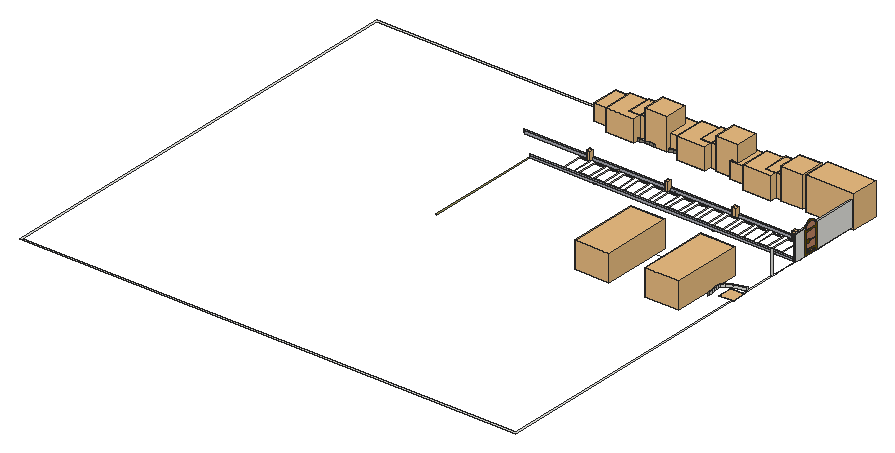
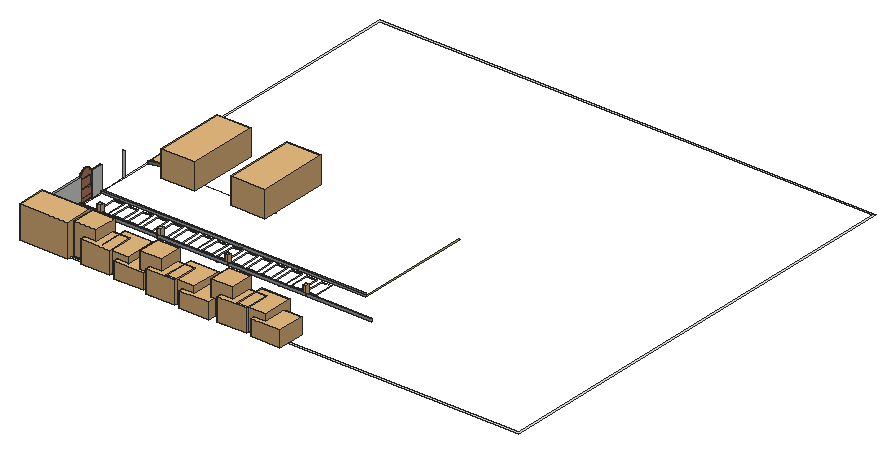
# SketchUp Ruby script. Lengths in inches.
U = 1.inch
M = Sketchup.active_model
def pt(a) = Geom::Point3d.new(a.map { |v| v * U })
def face(e, loops, mat)
  f = e.add_face(loops[0].map { |a| pt(a) })
  loops[1..].each { |l| e.add_face(l.map { |a| pt(a) }).erase! }
  f.material = f.back_material = mat if mat
  f
end
# faces: each face lists its corners as indices into pts; further lists are holes
def faces(e, pts, list, mat = nil) = list.each { |f| face(e, (f[0].is_a?(Array) ? f : [f]).map { |l| l.map { |i| pts[i] } }, mat) }
# xy, xz, yz: faces in a plane at the given z, y or x. An outline is a flat list of corners, or four numbers for a rectangle; further outlines are holes
def ring(l) = l.size == 4 ? [[l[0], l[1]], [l[2], l[1]], [l[2], l[3]], [l[0], l[3]]] : l.each_slice(2).to_a
def flat(e, list, mat, &to3) = list.each { |f| face(e, (f[0].is_a?(Array) ? f : [f]).map { |l| ring(l).map { |u, v| to3.(u, v) } }, mat) }
def xy(e, z, list, mat = nil) = flat(e, list, mat) { |x, y| [x, y, z] }
def xz(e, y, list, mat = nil) = flat(e, list, mat) { |x, z| [x, y, z] }
def yz(e, x, list, mat = nil) = flat(e, list, mat) { |y, z| [x, y, z] }
def lines(e, pts, list) = list.each { |a, b| e.add_line(pt(pts[a]), pt(pts[b])) }
# prism: a flat outline (further loops are holes) pulled along v
def prism(e, loops, v, mat = nil)
  f = face(e, loops, mat); d = Geom::Vector3d.new(v.map { |x| x * U })
  f.pushpull(f.normal.samedirection?(d) ? d.length : -d.length)
end
def box(e, o, s, mat = nil) = prism(e, [[o, [o[0] + s[0], o[1], o[2]], [o[0] + s[0], o[1] + s[1], o[2]], [o[0], o[1] + s[1], o[2]]]], [0, 0, s[2]], mat)
def at(x, y, z, deg = 0) = Geom::Transformation.translation(pt([x, y, z])) * Geom::Transformation.rotation(ORIGIN, Z_AXIS, deg.degrees)
def axes(o, x, y, z) = Geom::Transformation.new([*x, 0, *y, 0, *z, 0, *pt(o).to_a, 1])
def part(name) = M.definitions.add(name)
# library, detail: a bought-in or finely detailed component or shape, given as its bounding box
def library(name, o, s) = part(name).tap { |d| box(d.entities, o, s) }
def detail(e, o, s) = box(e.add_group.entities, o, s)
def put(e, d, t, mat = nil) = e.add_instance(d, t).tap { |i| i.material = mat if mat }
def group(e, t, mat = nil) = e.add_group.tap { |g| g.transformation = t; g.material = mat if mat }.entities
root = M.entities
M.materials.add("Marble_01_1K").color = [230, 221, 211]
M.materials.add("Marble_20_1K").color = [172, 173, 182]
M.materials.add("Material__4").color = [36, 36, 36]
M.materials.add("Material__6").color = [79, 108, 5]
M.materials.add("Plaster_06_1K").color = [141, 135, 122]
M.materials.add("Soil_04_1K").color = [152, 146, 88]
M.materials.add("[Color D08]").color = [102, 76, 0]
M.materials.add("[Modern Siding]").color = [191, 132, 100]
M.materials.add("calathea lutea").color = [121, 145, 80]
c1 = library("Group\#54",[0,0,0],[2062.46,2062.46,4833.66])
c2 = part("Landscape+Light")
put(c2.entities,c1,at(-2096.57,-1031.23,-3775.98))
c3 = library("ew",[-14.92,-16.84,0],[29.84,33.68,0.01])
c4 = part("Group\#156")
g1 = group(c4.entities,at(8.61,38.85,0))
xy(g1,0,[[0,0,2.82,19.1,22.58,0],[22.58,0,2.82,19.1,22.58,19.1]],"calathea lutea")
p = [[2.82,19.1,0],[7.19,48.22,5.13],[10.77,48.22,5.13],[12.74,48.22,5.13],[22.58,48.22,5.13],[22.58,19.1,0]]
faces(g1,p,[[0,1,2,3,4,5]],"calathea lutea")
g2 = group(c4.entities,at(-0.77,-7.77,0))
p = [[14.8125,23.31,1.46],[21.35,23.31,0],[14.8125,0,1.46],[21.35,0,0],[27.89,0,1.46],[27.89,23.31,1.46],
  [8.27,46.62,2.92],[21.35,46.62,0],[34.4375,46.62,2.92],[4.47,23.31,6.43],[0,0,8.59],[33.76,0,4.28],
  [33.76,23.31,4.28]]
faces(g2,p,[[0,1,2],[3,2,1],[4,3,5],[1,5,3],[6,7,0],[1,0,7],[5,1,8],[7,8,1],
  [9,0,2,10],[11,4,5,12],[9,6,0],[12,5,8]],"calathea lutea")
c5 = part("Group\#150")
xy(c5.entities,0,[[0,0,0,33.87,27.21,33.87,19.71,0]],"calathea lutea")
c6 = part("Group\#157")
xy(c6.entities,1.04,[[21.13,33.87,21.13,57.59,32.375,57.59,27.12,33.87]],"calathea lutea")
xy(c6.entities,1.32,[[0.12,33.87,7.74,57.59]],"calathea lutea")
p = [[7.74,33.87,1.32],[11.8,57.59,0.61],[15.24,57.59,0],[15.24,33.87,0],[18.43,57.59,0.5625],[21.13,57.59,1.04],
  [21.13,33.87,1.04],[15.24,77.7,2.36],[21.13,77.7,3.4],[7.74,57.59,1.32],[7.74,77.7,3.69],[36.83,77.7,3.4],
  [32.375,57.59,1.04],[0.12,57.59,1.32],[0.12,77.7,3.69]]
faces(c6.entities,p,[[0,1,2,3],[3,2,4],[3,4,5,6],[7,2,1],[8,4,2,7],[0,9,1],[7,1,9,10],[8,5,4],
  [11,12,5,8],[10,9,13,14]],"calathea lutea")
put(c6.entities,c5,axes([0,-16.9375,0],[1,0,0],[0,1.5,0],[0,0,1]))
c7 = part("Group\#155")
g3 = group(c7.entities,at(0,-17.3,0))
xy(g3,0,[[0,0,28.07,51.9]],"calathea lutea")
g4 = group(c7.entities,at(0.9,34.6,0))
xy(g4,0,[[13.14,0,13.14,26.22,16.85,26.22],[13.14,0,16.85,26.22,20.16,26.22,20.16,0]],"calathea lutea")
p = [[6.36,0,1.82],[9.95,26.22,0.86],[13.14,26.22,0],[13.14,0,0],[20.16,0,0],[20.16,26.22,0],
  [27.07,26.22,1.22],[27.07,0,1.22],[13.14,49.5625,5.91],[20.16,49.5625,5.91],[16.85,26.22,0],[27.07,49.5625,7.125],
  [6.36,26.22,1.82],[6.36,49.5625,7.72],[0,0,4.78],[0,26.22,4.78],[0,49.5625,10.6875]]
faces(g4,p,[[0,1,2,3],[4,5,6,7],[8,2,1],[9,10,2,8],[9,5,10],[11,6,5,9],[0,12,1],[8,1,12,13],
  [14,15,12,0],[13,12,15,16]],"calathea lutea")
c8 = part("Group\#154")
put(c8.entities,c5,axes([0,-16.9375,0],[1,0,0],[0,1.5,0],[0,0,1]))
g5 = group(c8.entities,at(-0.23,33.4,-0.35))
p = [[15.12,39.14,-19.87],[15.12,20.54,-11.86],[11.68,20.84,-11.33],[21.02,39.66,-18.97],[18.3125,20.82,-11.37],[7.62,21.2,-10.71],
  [7.62,39.8,-18.72],[21.02,21.06,-10.96],[36.72,39.66,-18.97],[32.26,21.06,-10.96],[0,21.2,-10.71],[0,39.8,-18.72],
  [7.62,0.66,1.15],[15.12,0,0],[21.02,0.52,0.9],[27.01,0.52,0.9],[0,0.66,1.15]]
faces(g5,p,[[0,1,2],[3,4,1,0],[0,2,5,6],[3,7,4],[8,9,7,3],[6,5,10,11],[12,2,1,13],[13,1,4],
  [13,4,7,14],[12,5,2],[14,7,9,15],[16,10,5,12]],"calathea lutea")
c9 = part("Foliage cluster")
put(c9.entities,c4,axes([37.24,8.07,75.17],[1,0,0],[0,0.45554,-0.89021],[0,0.89021,0.45554]))
put(c9.entities,c6,axes([69.44,65.48,16.68],[-0.53288,-0.84619,0],[0.14694,-0.09253,0.98481],[-0.83334,0.52478,0.17365]))
put(c9.entities,c7,axes([47.9375,70.43,17.04],[0.74664,-0.66523,0],[0.11552,0.12965,0.98481],[-0.65512,-0.7353,0.17365]))
put(c9.entities,c4,axes([76.19,10.66,75.17],[0.70711,0.70711,0],[-0.32212,0.32212,-0.89021],[-0.62948,0.62948,0.45554]))
put(c9.entities,c4,axes([101.91,40.03,75.17],[0,1,0],[-0.45554,0,-0.89021],[-0.89021,0,0.45554]))
put(c9.entities,c4,axes([99.32,78.99,75.17],[-0.70711,0.70711,0],[-0.32212,-0.32212,-0.89021],[-0.62948,-0.62948,0.45554]))
put(c9.entities,c7,axes([34.81,63.36,17.04],[0.99956,-0.02967,0],[0.00515,0.17357,0.98481],[-0.02922,-0.98437,0.17365]))
put(c9.entities,c7,axes([48,37.4,15.8],[-0.14436,0.98953,0],[-0.40248,-0.05871,0.91355],[0.90398,0.13188,0.40674]))
put(c9.entities,c6,axes([56.87,39.77,12.28],[-0.67695,0.4263,0],[-0.18016,-0.28609,0.72505],[0.38636,0.61353,0.33809]))
put(c9.entities,c6,axes([36.12,43.25,12.28],[0.18947,0.77724,0],[-0.32848,0.08007,0.72505],[0.70442,-0.17172,0.33809]))
put(c9.entities,c8,axes([35.1,54.93,11.375],[0.79719,0.06694,0],[-0.03636,0.43302,0.6717],[0.05621,-0.66934,0.43454]))
put(c9.entities,c6,axes([41.66,47.32,12.28],[0.45082,0.66088,0],[-0.2793,0.19053,0.72505],[0.59896,-0.40858,0.33809]))
put(c9.entities,c6,axes([47.89,59.4,12.28],[0.79719,0.06694,0],[-0.02829,0.33691,0.72505],[0.06067,-0.7225,0.33809]))
put(c9.entities,c8,axes([29.53,49.96,11.375],[0.65692,0.45657,0],[-0.248,0.35682,0.6717],[0.38335,-0.55156,0.43454]))
put(c9.entities,c8,axes([29.9,49.27,12.86],[0.34062,0.72386,0],[-0.22849,0.10752,0.7591],[0.68685,-0.32321,0.25252]))
put(c9.entities,c8,axes([36.33,48.82,8.99],[0.09232,0.62522,0],[-0.3396,0.05015,0.53064],[0.52495,-0.07752,0.34329]))
put(c9.entities,c8,axes([49.82,38.52,8.99],[-0.54622,0.31791,0],[-0.17268,-0.29669,0.53064],[0.26692,0.45862,0.34329]))
put(c9.entities,c8,axes([55.68,39.21,8.99],[-0.632,0.00221,0],[-0.0012,-0.34328,0.53064],[0.00185,0.53064,0.34329]))
c10 = library("Group\#28",[0,0,0],[86.94,78.77,46.4375])
c11 = library("Group\#14",[-978.71,-103.24,719.12],[90.2,76.4,68.29])
c12 = library("Group\#13",[-906.16,-138.28,686.8],[98.25,106.18,75.79])
c13 = library("Group\#202",[-3.47,-2.45,12.47],[53.14,54.93,75.51])
c14 = part("Group\#35")
put(c14.entities,c9,axes([161.54,39.59,6.01],[0.19523,-0.19694,0],[0.19694,0.19523,0],[0,0,0.24957]))
put(c14.entities,c10,axes([0,18.48,0.92],[0.83,0,0],[0,0.83,0],[0,0,0.83]))
put(c14.entities,c11,axes([859.63,98.87,-568.1],[0.79,0,0],[0,0.79,0],[0,0,0.79]),"Material__4")
put(c14.entities,c12,axes([669.69,95.42,-472.48],[0.69,0,0],[0,0.69,0],[0,0,0.69]),"Material__6")
put(c14.entities,c13,at(133.52,12.51,-9.6))
c15 = library("t1",[-17.79,-17.21,0],[35.58,34.42,0.01])
c16 = library("light",[-4,-4,0],[8,8,0.01])
c17 = library("tt",[-12.4,-12.1,0],[24.8,24.2,0.01])
c18 = library("Evoque+Azul+Marinho+As+Novinha+Fica+Loca+2017",[-10.19,-69.08,0],[168.96,82.02,63.04])
c19 = library("Group\#32",[86.45,10.0625,0],[116.41,67.6,78.39])
box(root,[1204.46,846.16,0],[4,28.07,60])
xy(root,0,[[8.46,0.95,8.46,1080.74,1208.46,1080.74,1208.46,918.16,1207.93,910.21,1204.99,910.21,1204.46,918.16,1204.46,1076.74,12.46,1076.74,12.46,4.95,1204.46,4.95,1204.46,703.68,1204.54,706.84,1204.46,706.82,1204.46,777.17,1208.46,777.17,1208.46,0.95],[1204.46,703.68,1204.46,706.82,1204.54,706.84],[1202.44,846.16,1202.44,918.16,1204.46,918.16,1204.46,910.21,1204.99,910.21,1206.46,888.16,1207.93,910.21,1206.46,888.16,1204.46,858.17,1205.06,846.16],[1202.44,846.16,1202.44,918.16,1204.46,918.16,1204.46,910.21,1204.99,910.21,1206.46,888.16,1208.46,858.17,1208.46,918.16,1206.46,888.16,1204.46,858.17,1205.06,846.16],[1205.06,846.16,1207.87,846.16,1208.46,858.17,1204.46,858.17],
  [1207.87,846.16,1208.46,846.16,1208.46,858.17],[1204.46,858.17,1206.46,888.16,1208.46,858.17],[1208.46,858.17,1206.46,888.16,1207.93,910.21,1208.46,910.21],[1206.46,888.16,1204.99,910.21,1207.93,910.21],[1204.46,910.21,1204.46,918.16,1204.99,910.21],
  [1207.93,910.21,1208.46,918.16,1208.46,910.21]])
xy(root,0,[[561.69,565.82,561.69,850.66,1202.44,850.66,1202.44,846.16,566.19,846.16,566.19,565.82]],"Soil_04_1K")
xz(root,777.17,[[1204.46,0,1208.46,60]])
xz(root,846.16,[[566.19,0,870.83,6],[870.83,0,1202.44,6]],"Marble_20_1K")
xz(root,850.66,[[561.69,0,870.83,6],[870.83,0,1202.44,6]],"Marble_20_1K")
xz(root,858.14,[[782.43,0,806.43,2],[818.43,0,842.43,2],[854.43,0,878.43,2],[890.43,0,914.43,2],[926.43,0,950.43,2],
  [962.43,0,986.43,2],[998.43,0,1022.43,2],[1034.43,0,1058.43,2]])
xz(root,858.14,[[638.43,0,662.43,2],[674.43,0,698.43,2],[710.43,0,734.43,2],[746.43,0,770.43,2],[1070.43,0,1094.43,2],
  [1106.43,0,1130.43,2],[1142.43,0,1166.43,2]],"Marble_01_1K")
xz(root,906.14,[[638.43,0,662.43,2],[674.43,0,698.43,2],[710.43,0,734.43,2],[746.43,0,770.43,2],[782.43,0,806.43,2],
  [818.43,0,842.43,2],[854.43,0,878.43,2],[890.43,0,914.43,2],[926.43,0,950.43,2],[962.43,0,986.43,2],
  [998.43,0,1022.43,2],[1034.43,0,1058.43,2],[1070.43,0,1094.43,2],[1106.43,0,1130.43,2],[1142.43,0,1166.43,2]],"Marble_01_1K")
xz(root,910.21,[[1204.46,0,1208.46,60]])
xz(root,913.66,[[498.69,0,1202.44,6]],"Marble_20_1K")
xz(root,918.16,[[494.19,0,1202.44,6]],"Marble_20_1K")
yz(root,638.43,[[858.14,0,906.14,2]],"Marble_01_1K")
yz(root,662.43,[[858.14,0,906.14,2]],"Marble_01_1K")
yz(root,674.43,[[858.14,0,906.14,2]],"Marble_01_1K")
yz(root,698.43,[[858.14,0,906.14,2]],"Marble_01_1K")
yz(root,710.43,[[858.14,0,906.14,2]],"Marble_01_1K")
yz(root,734.43,[[858.14,0,906.14,2]],"Marble_01_1K")
yz(root,746.43,[[858.14,0,906.14,2]],"Marble_01_1K")
yz(root,770.43,[[858.14,0,906.14,2]],"Marble_01_1K")
yz(root,782.43,[[858.14,0,906.14,2]],"Marble_01_1K")
yz(root,806.43,[[858.14,0,906.14,2]],"Marble_01_1K")
yz(root,818.43,[[858.14,0,906.14,2]])
yz(root,842.43,[[858.14,0,906.14,2]],"Marble_01_1K")
yz(root,854.43,[[858.14,0,906.14,2]],"Marble_01_1K")
yz(root,878.43,[[858.14,0,906.14,2]],"Marble_01_1K")
yz(root,890.43,[[858.14,0,906.14,2]],"Marble_01_1K")
yz(root,914.43,[[858.14,0,906.14,2]],"Marble_01_1K")
yz(root,926.43,[[858.14,0,906.14,2]],"Marble_01_1K")
yz(root,950.43,[[858.14,0,906.14,2]],"Marble_01_1K")
yz(root,962.43,[[858.14,0,906.14,2]],"Marble_01_1K")
yz(root,986.43,[[858.14,0,906.14,2]],"Marble_01_1K")
yz(root,998.43,[[858.14,0,906.14,2]],"Marble_01_1K")
yz(root,1022.43,[[858.14,0,906.14,2]],"Marble_01_1K")
yz(root,1034.43,[[858.14,0,906.14,2]],"Marble_01_1K")
yz(root,1058.43,[[858.14,0,906.14,2]],"Marble_01_1K")
yz(root,1070.43,[[858.14,0,906.14,2]],"Marble_01_1K")
yz(root,1094.43,[[858.14,0,906.14,2]],"Marble_01_1K")
yz(root,1106.43,[[858.14,0,906.14,2]],"Marble_01_1K")
yz(root,1130.43,[[858.14,0,906.14,2]],"Marble_01_1K")
yz(root,1142.43,[[858.14,0,906.14,2]],"Marble_01_1K")
yz(root,1166.43,[[858.14,0,906.14,2]],"Marble_01_1K")
yz(root,1202.44,[[846.16,0,850.66,6],[913.66,0,918.16,6]],"Soil_04_1K")
yz(root,1204.46,[[910.21,0,1063.52,60],[1063.52,0,1067.35,6],[1067.35,0,1076.74,60]])
yz(root,1208.46,[[910.21,0,1080.74,60]])
p = [[1157.58,649.72,0],[1158.71,642.73,0],[1158.71,642.73,6],[1157.58,649.72,6],[1160.94,646.1875,0],[1159.83,653.25,0],
  [1159.83,653.25,6],[1160.94,646.1875,6],[1156.54,656.72,0],[1156.54,656.72,6],[1158.82,660.32,0],[1158.82,660.32,6],
  [1155.61,663.74,0],[1155.61,663.74,6],[1157.94,667.38,0],[1157.94,667.38,6],[1154.79,670.79,0],[1154.79,670.79,6],
  [1157.2,674.44,0],[1157.2,674.44,6],[1154.1,677.86,0],[1154.1,677.86,6],[1157.46,681.53,0],[1157.46,681.53,6],
  [1154.57,684.97,0],[1154.57,684.97,6],[1162.47,688.71,0],[1162.47,688.71,6],[1160.14,692.15,0],[1160.14,692.15,6],
  [1176.67,696.07,0],[1176.67,696.07,6],[1175.31,699.43,0],[1175.31,699.43,6],[1204.46,703.68,0],[1204.46,703.68,6],
  [1204.46,706.82,0],[1204.54,706.84,6],[1204.54,706.84,0],[676.95,1026.38,0],[688.1,1026.27,0],[688.1,1026.27,6],
  [676.95,1026.38,6],[699.26,1026.43,0],[699.26,1026.43,6],[665.83,1026.8125,0],[665.83,1026.8125,6],[710.43,1026.85,0],
  [710.43,1026.85,6],[654.73,1027.59,0],[654.73,1027.59,6],[721.625,1027.5,0],[721.625,1027.5,6],[732.83,1028.35,0],
  [732.83,1028.35,6],[643.65,1028.72,0],[643.65,1028.72,6],[744.04,1029.36,0],[744.04,1029.36,6],[632.59,1030.19,0],
  [632.59,1030.19,6],[685.6,1029.27,0],[674.92,1029.4375,0],[674.92,1029.4375,6],[685.6,1029.27,6],[696.31,1029.36,0],
  [696.31,1029.36,6],[664.26,1029.91,0],[664.26,1029.91,6],[707.04,1029.7,0],[707.04,1029.7,6],[755.26,1030.51,0],
  [755.26,1030.51,6],[717.79,1030.26,0],[717.79,1030.26,6],[653.625,1030.7,0],[653.625,1030.7,6],[728.57,1031.01,0],
  [728.57,1031.01,6],[766.49,1031.78,0],[766.49,1031.78,6],[643.01,1031.82,0],[643.01,1031.82,6],[1075.29,1031.01,0],
  [1087.86,1030.73,0],[1087.86,1030.73,6],[1075.29,1031.01,6],[1100.42,1030.875,0],[1100.42,1030.875,6],[1112.91,1031.52,0],
  [1112.91,1031.52,6],[739.36,1031.93,0],[739.36,1031.93,6],[1062.76,1031.64,0],[1062.76,1031.64,6],[1125.29,1032.74,0],
  [1125.29,1032.74,6],[1050.3125,1032.55,0],[1050.3125,1032.55,6],[777.72,1033.12,0],[777.72,1033.12,6],[750.16,1032.99,0],
  [750.16,1032.99,6],[1038.01,1033.66,0],[1038.01,1033.66,6],[1137.5,1034.61,0],[1137.5,1034.61,6],[760.98,1034.16,0],
  [760.98,1034.16,6],[788.95,1034.52,0],[788.95,1034.52,6],[1025.89,1034.91,0],[1025.89,1034.91,6],[1094.48,1033.75,0],
  [1082.43,1033.8,0],[1082.43,1033.8,6],[1094.48,1033.75,6],[1106.47,1034.125,0],[1106.47,1034.125,6],[1070.375,1034.22,0],
  [1070.375,1034.22,6],[1118.36,1035,0],[1118.36,1035,6],[771.8125,1035.43,0],[771.8125,1035.43,6],[1058.36,1034.9375,0],
  [1058.36,1034.9375,6],[800.1875,1035.9375,0],[800.1875,1035.9375,6],[1149.5,1037.2,0],[1149.5,1037.2,6],[1013.97,1036.24,0],
  [1013.97,1036.24,6],[1046.43,1035.89,0],[1046.43,1035.89,6],[1130.1,1036.43,0],[1130.1,1036.43,6],[782.65,1036.75,0],
  [782.65,1036.75,6],[811.42,1037.35,0],[811.42,1037.35,6],[1034.625,1037.02,0],[1034.625,1037.02,6],[1002.24,1037.6,0],
  [1002.24,1037.6,6],[1141.65,1038.48,0],[1141.65,1038.48,6],[793.5,1038.11,0],[793.5,1038.11,6],[1023,1038.25,0],
  [1023,1038.25,6],[1161.22,1040.58,0],[1161.22,1040.58,6],[822.65,1038.73,0],[822.65,1038.73,6],[990.67,1038.95,0],
  [990.67,1038.95,6],[804.36,1039.49,0],[804.36,1039.49,6],[1011.54,1039.54,0],[1011.54,1039.54,6],[1152.96,1041.21,0],
  [1152.96,1041.21,6],[833.875,1040.05,0],[833.875,1040.05,6],[979.23,1040.27,0],[979.23,1040.27,6],[815.22,1040.85,0],
  [815.22,1040.85,6],[1000.25,1040.85,0],[1000.25,1040.85,6],[845.09,1041.27,0],[845.09,1041.27,6],[967.9,1041.5,0],
  [967.9,1041.5,6],[1172.64,1044.83,0],[1172.64,1044.83,6],[826.09,1042.16,0],[826.09,1042.16,6],[989.09,1042.16,0],
  [989.09,1042.16,6],[1163.99,1044.7,0],[1163.99,1044.7,6],[856.3,1042.37,0],[856.3,1042.37,6],[956.67,1042.61,0],
  [956.67,1042.61,6],[836.95,1043.41,0],[836.95,1043.41,6],[978.04,1043.42,0],[978.04,1043.42,6],[867.5,1043.32,0],
  [867.5,1043.32,6],[945.5,1043.55,0],[945.5,1043.55,6],[878.68,1044.1,0],[878.68,1044.1,6],[847.82,1044.57,0],
  [847.82,1044.57,6],[967.08,1044.6,0],[967.08,1044.6,6],[934.37,1044.3,0],[934.37,1044.3,6],[889.85,1044.66,0],
  [889.85,1044.66,6],[923.26,1044.8125,0],[923.26,1044.8125,6],[858.68,1045.6,0],[858.68,1045.6,6],[956.2,1045.66,0],
  [956.2,1045.66,6],[901.01,1044.99,0],[901.01,1044.99,6],[1174.69,1048.99,0],[1174.69,1048.99,6],[912.14,1045.04,0],
  [912.14,1045.04,6],[1183.68,1050.02,0],[1183.68,1050.02,6],[869.55,1046.49,0],[869.55,1046.49,6],[945.36,1046.57,0],
  [945.36,1046.57,6],[880.4,1047.2,0],[880.4,1047.2,6],[934.55,1047.3,0],[934.55,1047.3,6],[891.25,1047.72,0],
  [891.25,1047.72,6],[923.74,1047.8,0],[923.74,1047.8,6],[902.09,1048,0],[902.09,1048,6],[912.93,1048.04,0],
  [912.93,1048.04,6],[1185.03,1054.16,0],[1185.03,1054.16,6],[1194.31,1056.22,0],[1194.31,1056.22,6],[1194.96,1060.26,0],
  [1194.96,1060.26,6],[1204.46,1063.52,0],[1204.46,1063.52,6],[1204.46,1067.35,0],[1204.46,1067.35,6],[1147.61,704.82,0],
  [1111.7,704.82,0],[1208.46,777.17,0],[1206.46,817.67,0],[967.83,704.82,0],[931.7,704.82,0],[1057.72,704.82,0],
  [1021.59,704.82,0],[1075.57,704.82,0],[1207.87,846.16,0],[1205.06,846.16,0],[1204.46,777.17,0],[985.68,704.82,0],
  [895.78,704.82,0]]
faces(root,p,[[0,1,2,3],[8,0,3,9],[12,8,9,13],[16,12,13,17],[20,16,17,21],[24,20,21,25],[28,24,25,29],[32,28,29,33],
  [36,32,33,37,38],[39,40,41,42],[40,43,44,41],[45,39,42,46],[43,47,48,44],[49,45,46,50],[47,51,52,48],[51,53,54,52],
  [55,49,50,56],[53,57,58,54],[59,55,56,60],[57,71,72,58],[71,79,80,72],[83,84,85,86],[84,87,88,85],[87,89,90,88],
  [93,83,86,94],[89,95,96,90],[97,93,94,98],[79,99,100,80],[103,97,98,104],[95,105,106,96],[99,109,110,100],[111,103,104,112],
  [109,127,128,110],[105,129,130,106],[131,111,112,132],[127,139,140,128],[143,131,132,144],[129,151,152,130],[139,153,154,140],[155,143,144,156],
  [153,163,164,154],[165,155,156,166],[163,171,172,164],[173,165,166,174],[151,175,176,152],[171,183,184,172],[185,173,174,186],[183,191,192,184],
  [193,185,186,194],[191,195,196,192],[201,193,194,202],[195,203,204,196],[205,201,202,206],[203,211,212,204],[215,205,206,216],[175,217,218,176],
  [211,215,216,212],[217,237,238,218],[237,241,242,238]],"Plaster_06_1K")
faces(root,p,[[4,5,6,7],[5,10,11,6],[10,14,15,11],[14,18,19,15],[18,22,23,19],[22,26,27,23],[26,30,31,27],[30,34,35,31],
  [34,38,37,35],[61,62,63,64],[65,61,64,66],[62,67,68,63],[69,65,66,70],[73,69,70,74],[67,75,76,68],[77,73,74,78],
  [75,81,82,76],[91,77,78,92],[101,91,92,102],[107,101,102,108],[113,114,115,116],[117,113,116,118],[114,119,120,115],[121,117,118,122],
  [123,107,108,124],[119,125,126,120],[125,133,134,126],[135,121,122,136],[137,123,124,138],[133,141,142,134],[145,135,136,146],[147,137,138,148],
  [141,149,150,142],[157,147,148,158],[149,159,160,150],[161,145,146,162],[167,157,158,168],[159,169,170,160],[177,167,168,178],[169,179,180,170],
  [181,161,162,182],[187,177,178,188],[179,189,190,180],[197,187,188,198],[189,199,200,190],[207,197,198,208],[199,209,210,200],[213,181,182,214],
  [219,207,208,220],[209,221,222,210],[223,219,220,224],[221,225,226,222],[227,223,224,228],[225,229,230,226],[231,227,228,232],[229,233,234,230],
  [233,231,232,234],[235,213,214,236],[239,235,236,240],[243,239,240,244]])
lines(root,p,[[245,246],[247,248],[249,250],[251,252],[246,253],[254,248],[248,255],[248,256],[252,257],[253,251],[257,249],[250,258]])
put(root,c2,axes([662.46,912.36,16.63],[0.0044,0,0],[0,0.0044,0],[0,0,0.0044]))
put(root,c3,at(659.55,1050.15,0,90))
put(root,c14,at(568.58,1017.59,-3))
put(root,c15,at(703.79,1052.3,0,90))
put(root,c16,at(722.43,850.3,0))
put(root,c16,at(722.43,913.8,0))
put(root,c17,at(741.88,1051.8125,0,90))
put(root,c3,at(778.32,1050.15,0,90))
put(root,c15,at(822.5625,1052.3,0,90))
put(root,c14,at(740.8,1017.59,-3))
put(root,c2,axes([851.42,912.36,16.63],[0.0044,0,0],[0,0.0044,0],[0,0,0.0044]))
put(root,c17,at(859.96,1051.8125,0,90))
put(root,c16,at(866.43,850.3,0))
put(root,c16,at(866.43,913.8,0))
put(root,c3,at(896.4,1050.15,0,90))
put(root,c15,at(940.64,1052.3,0,90))
put(root,c18,axes([969.13,574.84,0],[0,1,0],[1,0,0],[0,0,1]))
put(root,c17,at(975.16,1051.8125,0,90))
put(root,c2,axes([1014.85,912.36,16.63],[0.0044,0,0],[0,0.0044,0],[0,0,0.0044]))
put(root,c14,at(908.76,1004.92,-3))
put(root,c16,at(1010.43,850.3,0))
put(root,c16,at(1010.43,913.8,0))
put(root,c3,at(1011.6,1050.15,0,90))
put(root,c15,at(1055.84,1052.3,0,90))
put(root,c17,at(1083.21,1051.8125,0,90))
put(root,c18,axes([1137.54,574.84,0],[0,1,0],[1,0,0],[0,0,1]))
put(root,c3,at(1119.65,1050.15,0,90))
put(root,c16,at(1154.43,850.3,0))
put(root,c16,at(1154.43,913.8,0))
put(root,c19,at(1010.61,1004.92,-3))
put(root,c2,axes([1160.54,912.36,16.63],[0.0044,0,0],[0,0.0044,0],[0,0,0.0044]))
put(root,c15,at(1163.89,1052.3,0,90))
put(root,c15,axes([1193.17,673.36,0],[1,0,0],[0,-1,0],[0,0,1]))
g6 = group(root,at(1206.46,874.23,0))
xy(g6,0,[[0,0,2,36]],"[Color D08]")
xy(g6,2.01,[[0,1.5,2,34.5]],"[Color D08]")
xy(g6,8.55,[[0,1.5,2,34.5]],"[Color D08]")
xy(g6,10.56,[[0,1.5,2,34.5]],"[Color D08]")
xy(g6,25.39,[[0,1.5,2,11.5]],"[Color D08]")
xy(g6,28.03,[[0,11.5,2,34.5]],"[Color D08]")
xy(g6,29.79,[[0,11.5,2,34.5]],"[Color D08]")
xy(g6,32.43,[[0,1.5,2,11.5]],"[Color D08]")
xy(g6,50.78,[[0,1.5,2,34.5]],"[Color D08]")
xy(g6,52.79,[[0,1.5,2,34.5]],"[Color D08]")
xz(g6,0,[[0,0,2,60.33]],"[Color D08]")
xz(g6,1.5,[[0,2.01,2,8.55],[0,10.56,2,25.39],[0,25.39,2,29.79],[0,29.79,2,32.43],[0,32.43,2,50.78],
  [0,52.79,2,59.58]],"[Color D08]")
xz(g6,11.5,[[0,25.39,2,28.03],[0,29.79,2,32.43]],"[Color D08]")
xz(g6,34.5,[[0,2.01,2,8.55],[0,8.55,2,10.56],[0,10.56,2,28.03],[0,28.03,2,50.78],[0,50.78,2,52.79],
  [0,52.79,2,59.58]],"[Color D08]")
xz(g6,36,[[0,0,2,60.33]],"[Color D08]")
yz(g6,0,[[[0,0,0,60.33,2.29,63.83,4.96,66.82,7.9375,69.22,11.16,70.97,14.54,72.04,18,72.4,21.46,72.04,24.84,70.97,28.0625,69.22,31.04,66.82,33.71,63.83,36,60.33,36,0],[1.5,10.56,34.5,50.78],[1.5,52.79,34.5,52.79,34.5,59.58,32.66,62.39,30.17,65.17,27.39,67.41,24.39,69.05,21.23,70.05,18,70.38,14.77,70.05,11.61,69.05,8.61,67.41,5.83,65.17,3.34,62.39,1.5,59.58],[1.5,2.01,34.5,8.55]],[1.5,29.79,11.5,32.43]],"[Color D08]")
yz(g6,0,[[1.5,2.01,34.5,8.55],[1.5,10.56,1.5,25.39,11.5,25.39,11.5,28.03,34.5,28.03,34.5,10.56],[1.5,25.39,1.5,29.79,34.5,29.79,34.5,28.03,11.5,28.03,11.5,25.39],[11.5,29.79,11.5,32.43,1.5,32.43,1.5,50.78,34.5,50.78,34.5,29.79],[1.5,52.79,34.5,52.79,34.5,59.58,32.66,62.39,30.17,65.17,27.39,67.41,24.39,69.05,21.23,70.05,18,70.38,14.77,70.05,11.61,69.05,8.61,67.41,5.83,65.17,3.34,62.39,1.5,59.58]],"[Modern Siding]")
yz(g6,2,[[[0,0,36,0,36,60.33,33.71,63.83,31.04,66.82,28.0625,69.22,24.84,70.97,21.46,72.04,18,72.4,14.54,72.04,11.16,70.97,7.9375,69.22,4.96,66.82,2.29,63.83,0,60.33],[1.5,10.56,34.5,50.78],[1.5,52.79,1.5,59.58,3.34,62.39,5.83,65.17,8.61,67.41,11.61,69.05,14.77,70.05,18,70.38,21.23,70.05,24.39,69.05,27.39,67.41,30.17,65.17,32.66,62.39,34.5,59.58,34.5,52.79],[1.5,2.01,34.5,8.55]],[1.5,25.39,11.5,25.39,11.5,28.03,34.5,28.03,34.5,29.79,11.5,29.79,11.5,32.43,1.5,32.43]],"[Color D08]")
p = [[0,1.5,59.58],[0,3.34,62.39],[2,3.34,62.39],[2,1.5,59.58],[0,32.66,62.39],[0,34.5,59.58],
  [2,34.5,59.58],[2,32.66,62.39],[0,2.29,63.83],[0,0,60.33],[2,0,60.33],[2,2.29,63.83],
  [0,36,60.33],[0,33.71,63.83],[2,33.71,63.83],[2,36,60.33],[0,5.83,65.17],[2,5.83,65.17],
  [0,30.17,65.17],[2,30.17,65.17],[0,4.96,66.82],[2,4.96,66.82],[0,31.04,66.82],[2,31.04,66.82],
  [0,8.61,67.41],[2,8.61,67.41],[0,27.39,67.41],[2,27.39,67.41],[0,7.9375,69.22],[2,7.9375,69.22],
  [0,28.0625,69.22],[2,28.0625,69.22],[0,11.61,69.05],[2,11.61,69.05],[0,24.39,69.05],[2,24.39,69.05],
  [0,14.77,70.05],[2,14.77,70.05],[0,21.23,70.05],[2,21.23,70.05],[0,11.16,70.97],[2,11.16,70.97],
  [0,24.84,70.97],[2,24.84,70.97],[0,18,70.38],[2,18,70.38],[0,14.54,72.04],[2,14.54,72.04],
  [0,21.46,72.04],[2,21.46,72.04],[0,18,72.4],[2,18,72.4]]
faces(g6,p,[[0,1,2,3],[4,5,6,7],[8,9,10,11],[12,13,14,15],[1,16,17,2],[18,4,7,19],[20,8,11,21],[13,22,23,14],
  [16,24,25,17],[26,18,19,27],[28,20,21,29],[22,30,31,23],[24,32,33,25],[34,26,27,35],[32,36,37,33],[38,34,35,39],
  [40,28,29,41],[30,42,43,31],[36,44,45,37],[44,38,39,45],[46,40,41,47],[42,48,49,43],[50,46,47,51],[48,50,51,49]],"[Color D08]")
